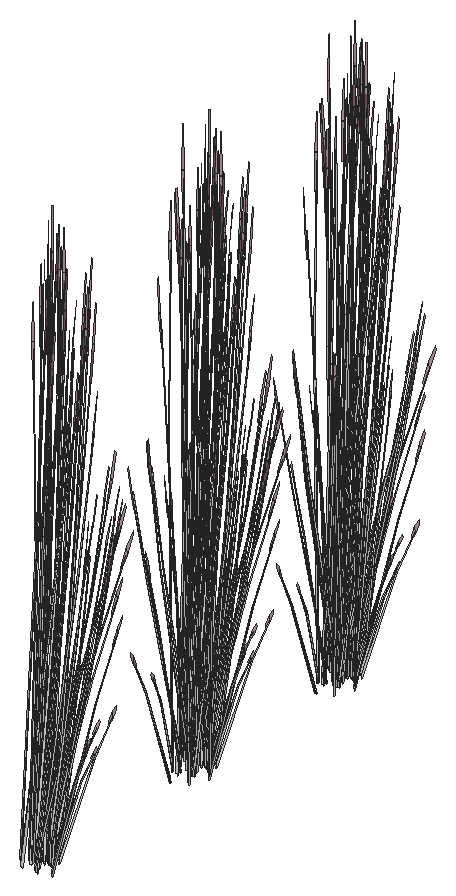
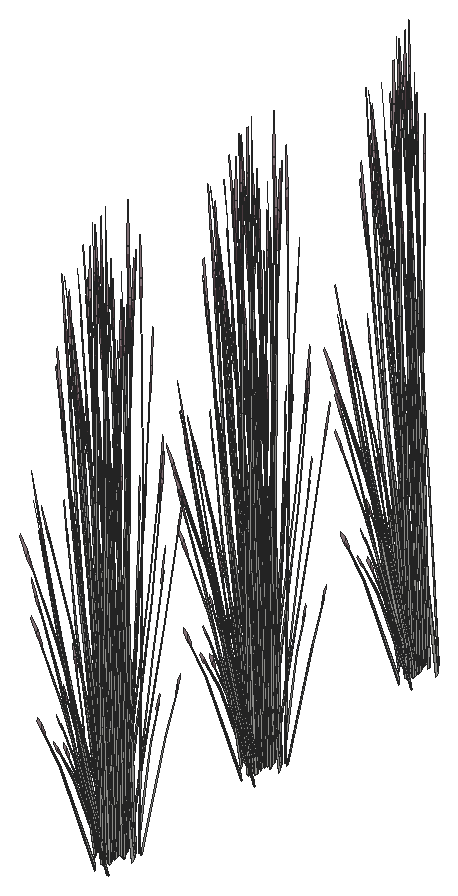
# SketchUp Ruby script. Lengths in inches.
U = 1.inch
M = Sketchup.active_model
def pt(a) = Geom::Point3d.new(a.map { |v| v * U })
def face(e, loops, mat)
  f = e.add_face(loops[0].map { |a| pt(a) })
  loops[1..].each { |l| e.add_face(l.map { |a| pt(a) }).erase! }
  f.material = f.back_material = mat if mat
  f
end
# faces: each face lists its corners as indices into pts; further lists are holes
def faces(e, pts, list, mat = nil) = list.each { |f| face(e, (f[0].is_a?(Array) ? f : [f]).map { |l| l.map { |i| pts[i] } }, mat) }
# xy, xz, yz: faces in a plane at the given z, y or x. An outline is a flat list of corners, or four numbers for a rectangle; further outlines are holes
def ring(l) = l.size == 4 ? [[l[0], l[1]], [l[2], l[1]], [l[2], l[3]], [l[0], l[3]]] : l.each_slice(2).to_a
def flat(e, list, mat, &to3) = list.each { |f| face(e, (f[0].is_a?(Array) ? f : [f]).map { |l| ring(l).map { |u, v| to3.(u, v) } }, mat) }
def xy(e, z, list, mat = nil) = flat(e, list, mat) { |x, y| [x, y, z] }
def xz(e, y, list, mat = nil) = flat(e, list, mat) { |x, z| [x, y, z] }
def yz(e, x, list, mat = nil) = flat(e, list, mat) { |y, z| [x, y, z] }
def lines(e, pts, list) = list.each { |a, b| e.add_line(pt(pts[a]), pt(pts[b])) }
# prism: a flat outline (further loops are holes) pulled along v
def prism(e, loops, v, mat = nil)
  f = face(e, loops, mat); d = Geom::Vector3d.new(v.map { |x| x * U })
  f.pushpull(f.normal.samedirection?(d) ? d.length : -d.length)
end
def box(e, o, s, mat = nil) = prism(e, [[o, [o[0] + s[0], o[1], o[2]], [o[0] + s[0], o[1] + s[1], o[2]], [o[0], o[1] + s[1], o[2]]]], [0, 0, s[2]], mat)
def at(x, y, z, deg = 0) = Geom::Transformation.translation(pt([x, y, z])) * Geom::Transformation.rotation(ORIGIN, Z_AXIS, deg.degrees)
def axes(o, x, y, z) = Geom::Transformation.new([*x, 0, *y, 0, *z, 0, *pt(o).to_a, 1])
def part(name) = M.definitions.add(name)
# library, detail: a bought-in or finely detailed component or shape, given as its bounding box
def library(name, o, s) = part(name).tap { |d| box(d.entities, o, s) }
def detail(e, o, s) = box(e.add_group.entities, o, s)
def put(e, d, t, mat = nil) = e.add_instance(d, t).tap { |i| i.material = mat if mat }
def group(e, t, mat = nil) = e.add_group.tap { |g| g.transformation = t; g.material = mat if mat }.entities
root = M.entities
M.materials.add("LightPink_Translucent").color = [144, 107, 117]
M.materials["LightPink_Translucent"].alpha = 0.75
c1 = part("blade")
p = [[2.15,0.21,22],[0,0.17,0],[0.09,0.45,0],[2.18,0.31,22],[2.29,0.31,22],[0.38,0.45,0],
  [2.48,0.24,33],[2.49,0.24,33],[2.48,0.22,33]]
faces(c1.entities,p,[[0,1,2,3],[4,5,2,3],[6,3,4,7],[8,0,3,6]])
c2 = part("seeds")
p = [[0.3,-0.1,1.38],[-0.01,-0.03,1.59],[-0.01,-0.03,0.03],[0.14,-0.07,-0.07],[0.29,-0.03,3],[0.15,0.01,3.11]]
faces(c2.entities,p,[[0,1,2,3],[1,0,4,5]],"LightPink_Translucent")
c3 = part("blade with seeds")
put(c3.entities,c1,at(0,0,0))
put(c3.entities,c2,axes([2.4,0.25,30.99],[1.5799,-0.05474,1.17369],[-0.12525,1.92788,0.29478],[-0.07173,-0.02425,1.56792]))
put(root,c3,axes([403.51,539.17,4.98],[0.31014,-0.20596,-0.71045],[0.17284,0.42397,0.08574],[0.14985,-0.04816,1.00501]))
put(root,c3,axes([402.12,538.4375,2.36],[-0.29264,0.42323,0.45755],[-0.34767,-0.3736,0.17955],[0.07055,-0.04224,1.58856]))
put(root,c3,axes([401.61,537.74,2.47],[-0.10196,0.46348,0.17642],[-0.3731,-0.13116,0.35086],[0.06445,-0.00226,1.60407]))
put(root,c3,axes([401.46,538.11,1.59],[-0.3474,0.18671,1.28929],[-0.11057,-0.53572,0.50096],[0.21332,0.00891,1.46642]))
put(root,c3,axes([402.39,538.25,2.62],[0.06809,-0.4162,0.1448],[0.33266,0.07225,-0.41347],[0.06054,0.04274,1.26744]))
put(root,c3,axes([404.17,538.84,1.49],[-0.01845,-0.0708,1.76342],[0.12793,-0.41416,-0.26939],[0.12905,-0.00596,0.30037]))
put(root,c3,axes([402.25,538.36,2.72],[-0.21202,-0.39143,0.44739],[0.32115,-0.27564,-0.21531],[0.06861,0.04843,1.43643]))
put(root,c3,axes([402.36,538.39,2.67],[0.35635,-0.30962,-0.29095],[0.23697,0.43749,-0.50002],[0.08792,0.04443,1.59708]))
put(root,c3,axes([403.78,539.21,4.53],[0.29332,0.1301,-0.35414],[-0.08555,0.37955,0.4572],[0.11809,-0.0348,0.87481]))
put(root,c3,axes([403.26,537.57,2.02],[0.33032,0.23318,-0.49651],[-0.19744,0.41812,0],[0.07523,0.05311,1.57504]))
put(root,c3,axes([402.63,538.9,2.21],[0.39487,0,0],[0,0.48281,0],[0,0,1.78407]))
put(root,c3,axes([402.74,537.76,2.47],[-0.37926,0.12378,0.17642],[-0.09365,-0.46065,0.35086],[0.03382,0.06712,1.60407]))
put(root,c3,axes([402.98,538.74,3.875],[-0.14639,0.01056,1.71376],[0.09712,-0.45778,0.13857],[0.20862,0.02831,0.73262]))
put(root,c3,axes([403.17,537.74,2.03],[0.08291,0.40636,-0.30978],[-0.32928,0.11539,0.30978],[0.06638,0.04686,1.38974]))
put(root,c3,axes([402.5,538.65,2.38],[-0.44609,-0.09826,0.49198],[0.09078,-0.55493,0.19306],[0.06519,0.05359,1.70813]))
put(root,c3,axes([402.15,540.02,2.2],[-0.11516,-0.40207,0],[0.32884,-0.1408,0],[0,0,1.54371]))
put(root,c3,axes([402.58,539.96,2.18],[0.37054,-0.15823,-0.19198],[0.1302,0.45581,0.00008],[0.0409,-0.01749,1.73897]))
put(root,c3,axes([402.62,539.1,2.21],[0.24637,0.30123,0],[-0.24637,0.30123,0],[0,0,1.69266]))
put(root,c3,axes([403.29,538.97,2.47],[-0.2773,-0.3397,0.17642],[0.27945,-0.32949,0.35086],[-0.03063,0.06937,1.60407]))
put(root,c3,axes([402.78,538.46,2.06],[0.36714,0.07646,-0.62353],[-0.07747,0.47163,-0.16365],[0.10956,0.05715,1.37633]))
put(root,c3,axes([404.4,539.28,2.77],[-0.21807,0.07699,1.1486],[0.10265,-0.31819,0.84392],[0.11568,0.02177,0.25299]))
put(root,c3,axes([402.62,538.75,2.72],[0.17124,-0.42022,0.44739],[0.35581,0.20224,-0.21531],[0,0.09687,1.43643]))
put(root,c3,axes([402.55,538.99,2.29],[0,0.53934,-0.05637],[-0.44133,0,0],[0,0.01695,1.79368]))
put(root,c3,axes([402.58,538.61,2.21],[0.21202,0.39143,-0.44739],[-0.32115,0.27564,0.21531],[0.06861,0.04843,1.43643]))
put(root,c3,axes([404.02,540.26,3.93],[-0.06755,-0.39203,-0.03492],[0.31928,-0.09013,-0.15832],[0.06667,0.02485,0.52218]))
put(root,c3,axes([403.52,538.99,2.48],[0,-0.46636,0.49651],[0.39487,0,0],[0,0.10622,1.57504]))
put(root,c3,axes([402.77,538.85,2.62],[0.32884,-0.136,0.1448],[0.11516,0.38837,-0.41347],[0,0.08547,1.26744]))
put(root,c3,axes([403.99,539.79,2.59],[-0.085,-0.1147,1.43002],[0.1106,-0.37943,-0.30754],[0.17198,0.0514,0.61141]))
put(root,c3,axes([402.47,540.21,2.2],[0.35581,0.20937,0],[-0.17124,0.43505,0],[0,0,1.74954]))
put(root,c3,axes([403.21,540.02,4.98],[0.35281,0.01123,-0.71045],[-0.0237,0.47284,0.08574],[0.14947,0.0499,1.00501]))
put(root,c3,axes([402.8125,540.4,2.48],[0.33032,-0.23318,0.49651],[0.19744,0.41812,0],[-0.07523,0.05311,1.57504]))
put(root,c3,axes([402.34,540.04,2.29],[0.15345,0.53576,-0.06012],[-0.43845,0.18773,0],[0.00536,0.01871,1.72173]))
put(root,c3,axes([403.78,539.06,2.375],[0.44133,0,0],[0,0.52122,-0.51607],[0,0.11871,1.63711]))
put(root,c3,axes([403.61,539.33,2.2],[-0.44111,-0.00373,-0.04976],[0,-0.52122,0.49943],[-0.01386,0.11865,1.58352]))
put(root,c3,axes([402.65,538.88,2.67],[0.39748,0.22252,-0.29095],[-0.19139,0.46966,-0.50002],[0.01249,0.11531,1.59708]))
put(root,c3,axes([403.42,540.22,4.53],[0.20082,0.29199,-0.35414],[-0.2293,0.2764,0.4572],[0.1165,0.04206,0.87481]))
put(root,c3,axes([403.52,539.41,2.03],[-0.24637,0.29097,-0.30978],[-0.24637,-0.29097,0.30978],[0,0.09372,1.38974]))
put(root,c3,axes([402.61,539.23,2.21],[-0.17124,0.42022,-0.44739],[-0.35581,-0.20224,0.21531],[0,0.09687,1.43643]))
put(root,c3,axes([402.62,540.43,2.33],[0.44186,0.15158,0.30756],[-0.11054,0.54181,-0.36492],[-0.07313,0.06781,1.64885]))
put(root,c3,axes([403.6875,539.42,2.02],[0,0.46636,-0.49651],[-0.39487,0,0],[0,0.10622,1.57504]))
put(root,c3,axes([402.7,539.47,3.875],[-0.1311,-0.08035,1.71376],[0.27131,-0.33708,0.13857],[0.16909,0.15206,0.73262]))
put(root,c3,axes([403.18,540.39,2.77],[-0.19872,-0.13409,1.1486],[0.2566,-0.13625,0.84392],[0.06921,0.11541,0.25299]))
put(root,c3,axes([403.24,540.88,1.49],[0.02571,-0.06733,1.76342],[0.32373,-0.19829,-0.26939],[0.09815,0.10263,0.30037]))
put(root,c3,axes([402.8125,539.36,2.09],[0.12941,0.42699,-0.69212],[-0.37279,0.15378,-0.18165],[0.0143,0.14459,1.52773]))
put(root,c3,axes([402.74,540.57,4.68],[0.34827,-0.11086,-0.51099],[0.06092,0.41983,-0.3958],[0.09354,0.12031,0.97773]))
put(root,c3,axes([403.22,541,2.67],[-0.22633,-0.01463,1.0506],[0.14947,-0.31064,0.58006],[0.08941,0.11036,0.8241]))
put(root,c3,axes([402.48,540.24,2.59],[0.00623,-0.15459,1.43002],[0.29764,-0.17268,-0.30754],[0.09188,0.18503,0.61141]))
put(root,c3,axes([401.73,540.87,1.49],[0.05712,-0.02538,1.76342],[0.34359,0.13968,-0.26939],[0.01005,0.15742,0.30037]))
put(root,c3,axes([401.96,540.77,4.68],[0.34695,0.11691,-0.51099],[-0.11892,0.40083,-0.3958],[0.03181,0.16138,0.97773]))
put(root,c3,axes([402.16,539.9375,3.875],[-0.08068,-0.14973,1.71376],[0.3728,-0.12606,0.13857],[0.08426,0.23506,0.73262]))
put(root,c3,axes([401.8,541.01,4.53],[-0.1064,0.35863,-0.35414],[-0.31043,-0.1046,0.4572],[0.02846,0.14439,0.87481]))
put(root,c3,axes([401.84,540.6875,4.98],[0.16845,0.3792,-0.71045],[-0.34676,0.21133,0.08574],[0.03939,0.18322,1.00501]))
put(root,c3,axes([402.72,558.63,2.59],[-0.10032,0.0944,1.43002],[-0.30046,-0.16522,-0.30754],[0.05569,-0.20547,0.61141]))
put(root,c3,axes([401.98,558.12,1.49],[-0.0592,0.0168,1.76342],[-0.32738,-0.18913,-0.26939],[0.00549,-0.15776,0.30037]))
put(root,c3,axes([402.97,559.33,4.98],[0.00918,-0.43138,-0.71045],[0.38672,0.02897,0.08574],[0.04081,-0.18275,1.00501]))
put(root,c3,axes([402.3,558.64,4.53],[0.1064,-0.35863,-0.35414],[0.31043,0.1046,0.4572],[-0.02846,-0.14439,0.87481]))
put(root,c3,axes([402.53,559.12,3.875],[-0.06572,0.16029,1.71376],[-0.27569,-0.33172,0.13857],[0.12437,-0.20675,0.73262]))
put(root,c3,axes([402.35,557.88,2.77],[0.04528,0.27194,1.1486],[-0.25117,-0.15062,0.84392],[0.02703,-0.13924,0.25299]))
put(root,c3,axes([402.89,559.19,4.68],[-0.25266,-0.31335,-0.51099],[0.2669,-0.27442,-0.3958],[0.03844,-0.15921,0.97773]))
put(root,c3,axes([403.13,559.07,4.53],[0.23881,-0.24554,-0.35414],[0.22606,0.28036,0.4572],[0.0344,-0.14245,0.87481]))
put(root,c3,axes([403.43,558.93,1.49],[-0.05283,-0.03674,1.76342],[-0.13569,-0.41045,-0.26939],[0.09154,-0.11138,0.30037]))
put(root,c3,axes([403.42,560.08,4.98],[0.18436,-0.36797,-0.71045],[0.32306,0.26151,0.08574],[0.11008,-0.13332,1.00501]))
put(root,c3,axes([401.43,559.01,2.375],[-0.22066,-0.46731,0],[0.36918,-0.26061,-0.51607],[0.08408,-0.05936,1.63711]))
put(root,c3,axes([403.41,559.91,4.68],[-0.09067,-0.42583,-0.51099],[0.34336,-0.07449,-0.3958],[0.0984,-0.11438,0.97773]))
put(root,c3,axes([401.73,558.94,2.02],[0.33032,-0.23318,-0.49651],[0.19744,0.41812,0],[0.07523,-0.05311,1.57504]))
put(root,c3,axes([403.69,559.75,2.59],[-0.12609,-0.01381,1.43002],[-0.12917,-0.37055,-0.30754],[0.1549,-0.10482,0.61141]))
put(root,c3,axes([402.12,559.9,2.06],[0.23773,-0.35053,-0.62353],[0.29532,0.31785,-0.16365],[0.09526,-0.08744,1.37633]))
put(root,c3,axes([403.84,559.06,2.77],[-0.11756,0.2374,1.1486],[-0.10105,-0.31895,0.84392],[0.09709,-0.07992,0.25299]))
put(root,c3,axes([403.67,559.96,4.53],[0.30722,-0.06665,-0.35414],[0.08112,0.381,0.4572],[0.08804,-0.10234,0.87481]))
put(root,c3,axes([401.71,560.51,2.21],[0.17124,-0.42022,-0.44739],[0.35581,0.20224,0.21531],[0,-0.09687,1.43643]))
put(root,c3,axes([401.86,560.3,2.67],[-0.04113,-0.53214,-0.29095],[0.42835,-0.03218,-0.50002],[0.07543,-0.07088,1.59708]))
put(root,c3,axes([401.81,559.125,2.03],[0.32928,0.11539,-0.30978],[-0.08291,0.40636,0.30978],[0.06638,-0.04686,1.38974]))
put(root,c3,axes([401.92,560.72,2.43],[0.39767,0.22603,0.24065],[-0.19139,0.46966,0.50002],[0,-0.10827,1.60543]))
put(root,c3,axes([401.79,560.4,2.72],[-0.38326,0.02879,0.44739],[-0.03466,-0.47788,-0.21531],[0.06861,-0.04843,1.43643]))
put(root,c3,axes([403.57,560.86,4.68],[0.09562,-0.42421,-0.51099],[0.32782,0.1454,-0.3958],[0.13199,-0.0389,0.97773]))
put(root,c3,axes([403.06,559.13,2.375],[0.22066,-0.46731,0],[0.36918,0.26061,-0.51607],[0.08408,0.05936,1.63711]))
put(root,c3,axes([401.78,560.58,2.36],[0.15345,0.52148,0.45755],[-0.43845,0.18134,0.17955],[0.00536,-0.09582,1.58856]))
put(root,c3,axes([403.92,560.98,1.98],[-0.22732,0.05597,1.41583],[-0.03618,-0.44548,0.08104],[0.15921,-0.06743,0.80566]))
put(root,c3,axes([404.34,560.58,2.26],[-0.21881,-0.29821,-0.06488],[0.23965,-0.27324,-0.29416],[0.0679,-0.01924,0.97024]))
put(root,c3,axes([402.33,560.62,2.21],[0,-0.53961,0],[0.44133,0,0],[0,0,1.79456]))
put(root,c3,axes([402.87,559.375,2.48],[-0.33032,-0.23318,0.49651],[0.19744,-0.41812,0],[0.07523,0.05311,1.57504]))
put(root,c3,axes([403.51,561.01,4.98],[0.31014,-0.20596,-0.71045],[0.17284,0.42397,0.08574],[0.14985,-0.04816,1.00501]))
put(root,c3,axes([402.12,560.28,2.36],[-0.29264,0.42323,0.45755],[-0.34767,-0.3736,0.17955],[0.07055,-0.04224,1.58856]))
put(root,c3,axes([401.61,559.58,2.47],[-0.10196,0.46348,0.17642],[-0.3731,-0.13116,0.35086],[0.06445,-0.00226,1.60407]))
put(root,c3,axes([401.46,559.96,1.59],[-0.3474,0.18671,1.28929],[-0.11057,-0.53572,0.50096],[0.21332,0.00891,1.46642]))
put(root,c3,axes([402.39,560.1,2.62],[0.06809,-0.4162,0.1448],[0.33266,0.07225,-0.41347],[0.06054,0.04274,1.26744]))
put(root,c3,axes([404.17,560.6875,1.49],[-0.01845,-0.0708,1.76342],[0.12793,-0.41416,-0.26939],[0.12905,-0.00596,0.30037]))
put(root,c3,axes([402.25,560.21,2.72],[-0.21202,-0.39143,0.44739],[0.32115,-0.27564,-0.21531],[0.06861,0.04843,1.43643]))
put(root,c3,axes([402.36,560.23,2.67],[0.35635,-0.30962,-0.29095],[0.23697,0.43749,-0.50002],[0.08792,0.04443,1.59708]))
put(root,c3,axes([403.78,561.05,4.53],[0.29332,0.1301,-0.35414],[-0.08555,0.37955,0.4572],[0.11809,-0.0348,0.87481]))
put(root,c3,axes([403.26,559.41,2.02],[0.33032,0.23318,-0.49651],[-0.19744,0.41812,0],[0.07523,0.05311,1.57504]))
put(root,c3,axes([402.63,560.74,2.21],[0.39487,0,0],[0,0.48281,0],[0,0,1.78407]))
put(root,c3,axes([402.74,559.61,2.47],[-0.37926,0.12378,0.17642],[-0.09365,-0.46065,0.35086],[0.03382,0.06712,1.60407]))
put(root,c3,axes([402.98,560.58,3.875],[-0.14639,0.01056,1.71376],[0.09712,-0.45778,0.13857],[0.20862,0.02831,0.73262]))
put(root,c3,axes([403.17,559.59,2.03],[0.08291,0.40636,-0.30978],[-0.32928,0.11539,0.30978],[0.06638,0.04686,1.38974]))
put(root,c3,axes([402.5,560.5,2.38],[-0.44609,-0.09826,0.49198],[0.09078,-0.55493,0.19306],[0.06519,0.05359,1.70813]))
put(root,c3,axes([402.15,561.87,2.2],[-0.11516,-0.40207,0],[0.32884,-0.1408,0],[0,0,1.54371]))
put(root,c3,axes([402.58,561.81,2.18],[0.37054,-0.15823,-0.19198],[0.1302,0.45581,0.00008],[0.0409,-0.01749,1.73897]))
put(root,c3,axes([402.62,560.95,2.21],[0.24637,0.30123,0],[-0.24637,0.30123,0],[0,0,1.69266]))
put(root,c3,axes([403.29,560.82,2.47],[-0.2773,-0.3397,0.17642],[0.27945,-0.32949,0.35086],[-0.03063,0.06937,1.60407]))
put(root,c3,axes([402.78,560.3,2.06],[0.36714,0.07646,-0.62353],[-0.07747,0.47163,-0.16365],[0.10956,0.05715,1.37633]))
put(root,c3,axes([404.4,561.13,2.77],[-0.21807,0.07699,1.1486],[0.10265,-0.31819,0.84392],[0.11568,0.02177,0.25299]))
put(root,c3,axes([402.62,560.6,2.72],[0.17124,-0.42022,0.44739],[0.35581,0.20224,-0.21531],[0,0.09687,1.43643]))
put(root,c3,axes([402.55,560.84,2.29],[0,0.53934,-0.05637],[-0.44133,0,0],[0,0.01695,1.79368]))
put(root,c3,axes([402.58,560.45,2.21],[0.21202,0.39143,-0.44739],[-0.32115,0.27564,0.21531],[0.06861,0.04843,1.43643]))
put(root,c3,axes([404.02,562.11,3.93],[-0.06755,-0.39203,-0.03492],[0.31928,-0.09013,-0.15832],[0.06667,0.02485,0.52218]))
put(root,c3,axes([403.52,560.83,2.48],[0,-0.46636,0.49651],[0.39487,0,0],[0,0.10622,1.57504]))
put(root,c3,axes([402.77,560.69,2.62],[0.32884,-0.136,0.1448],[0.11516,0.38837,-0.41347],[0,0.08547,1.26744]))
put(root,c3,axes([403.99,561.64,2.59],[-0.085,-0.1147,1.43002],[0.1106,-0.37943,-0.30754],[0.17198,0.0514,0.61141]))
put(root,c3,axes([402.47,562.06,2.2],[0.35581,0.20937,0],[-0.17124,0.43505,0],[0,0,1.74954]))
put(root,c3,axes([403.21,561.87,4.98],[0.35281,0.01123,-0.71045],[-0.0237,0.47284,0.08574],[0.14947,0.0499,1.00501]))
put(root,c3,axes([402.8125,562.25,2.48],[0.33032,-0.23318,0.49651],[0.19744,0.41812,0],[-0.07523,0.05311,1.57504]))
put(root,c3,axes([402.34,561.88,2.29],[0.15345,0.53576,-0.06012],[-0.43845,0.18773,0],[0.00536,0.01871,1.72173]))
put(root,c3,axes([403.78,560.91,2.375],[0.44133,0,0],[0,0.52122,-0.51607],[0,0.11871,1.63711]))
put(root,c3,axes([403.61,561.18,2.2],[-0.44111,-0.00373,-0.04976],[0,-0.52122,0.49943],[-0.01386,0.11865,1.58352]))
put(root,c3,axes([402.65,560.72,2.67],[0.39748,0.22252,-0.29095],[-0.19139,0.46966,-0.50002],[0.01249,0.11531,1.59708]))
put(root,c3,axes([403.42,562.0625,4.53],[0.20082,0.29199,-0.35414],[-0.2293,0.2764,0.4572],[0.1165,0.04206,0.87481]))
put(root,c3,axes([403.52,561.25,2.03],[-0.24637,0.29097,-0.30978],[-0.24637,-0.29097,0.30978],[0,0.09372,1.38974]))
put(root,c3,axes([402.61,561.07,2.21],[-0.17124,0.42022,-0.44739],[-0.35581,-0.20224,0.21531],[0,0.09687,1.43643]))
put(root,c3,axes([402.62,562.28,2.33],[0.44186,0.15158,0.30756],[-0.11054,0.54181,-0.36492],[-0.07313,0.06781,1.64885]))
put(root,c3,axes([403.6875,561.26,2.02],[0,0.46636,-0.49651],[-0.39487,0,0],[0,0.10622,1.57504]))
put(root,c3,axes([402.7,561.32,3.875],[-0.1311,-0.08035,1.71376],[0.27131,-0.33708,0.13857],[0.16909,0.15206,0.73262]))
put(root,c3,axes([403.18,562.23,2.77],[-0.19872,-0.13409,1.1486],[0.2566,-0.13625,0.84392],[0.06921,0.11541,0.25299]))
put(root,c3,axes([403.24,562.73,1.49],[0.02571,-0.06733,1.76342],[0.32373,-0.19829,-0.26939],[0.09815,0.10263,0.30037]))
put(root,c3,axes([402.8125,561.2,2.09],[0.12941,0.42699,-0.69212],[-0.37279,0.15378,-0.18165],[0.0143,0.14459,1.52773]))
put(root,c3,axes([402.74,562.42,4.68],[0.34827,-0.11086,-0.51099],[0.06092,0.41983,-0.3958],[0.09354,0.12031,0.97773]))
put(root,c3,axes([403.22,562.84,2.67],[-0.22633,-0.01463,1.0506],[0.14947,-0.31064,0.58006],[0.08941,0.11036,0.8241]))
put(root,c3,axes([402.48,562.09,2.59],[0.00623,-0.15459,1.43002],[0.29764,-0.17268,-0.30754],[0.09188,0.18503,0.61141]))
put(root,c3,axes([401.73,562.71,1.49],[0.05712,-0.02538,1.76342],[0.34359,0.13968,-0.26939],[0.01005,0.15742,0.30037]))
put(root,c3,axes([401.96,562.61,4.68],[0.34695,0.11691,-0.51099],[-0.11892,0.40083,-0.3958],[0.03181,0.16138,0.97773]))
put(root,c3,axes([402.16,561.78,3.875],[-0.08068,-0.14973,1.71376],[0.3728,-0.12606,0.13857],[0.08426,0.23506,0.73262]))
put(root,c3,axes([401.8,562.86,4.53],[-0.1064,0.35863,-0.35414],[-0.31043,-0.1046,0.4572],[0.02846,0.14439,0.87481]))
put(root,c3,axes([401.84,562.53,4.98],[0.16845,0.3792,-0.71045],[-0.34676,0.21133,0.08574],[0.03939,0.18322,1.00501]))
put(root,c3,axes([402.72,578.9,2.59],[-0.10032,0.0944,1.43002],[-0.30046,-0.16522,-0.30754],[0.05569,-0.20547,0.61141]))
put(root,c3,axes([401.98,578.39,1.49],[-0.0592,0.0168,1.76342],[-0.32738,-0.18913,-0.26939],[0.00549,-0.15776,0.30037]))
put(root,c3,axes([402.97,579.6,4.98],[0.00918,-0.43138,-0.71045],[0.38672,0.02897,0.08574],[0.04081,-0.18275,1.00501]))
put(root,c3,axes([402.3,578.91,4.53],[0.1064,-0.35863,-0.35414],[0.31043,0.1046,0.4572],[-0.02846,-0.14439,0.87481]))
put(root,c3,axes([402.53,579.38,3.875],[-0.06572,0.16029,1.71376],[-0.27569,-0.33172,0.13857],[0.12437,-0.20675,0.73262]))
put(root,c3,axes([402.35,578.15,2.77],[0.04528,0.27194,1.1486],[-0.25117,-0.15062,0.84392],[0.02703,-0.13924,0.25299]))
put(root,c3,axes([402.89,579.46,4.68],[-0.25266,-0.31335,-0.51099],[0.2669,-0.27442,-0.3958],[0.03844,-0.15921,0.97773]))
put(root,c3,axes([403.13,579.34,4.53],[0.23881,-0.24554,-0.35414],[0.22606,0.28036,0.4572],[0.0344,-0.14245,0.87481]))
put(root,c3,axes([403.43,579.19,1.49],[-0.05283,-0.03674,1.76342],[-0.13569,-0.41045,-0.26939],[0.09154,-0.11138,0.30037]))
put(root,c3,axes([403.42,580.35,4.98],[0.18436,-0.36797,-0.71045],[0.32306,0.26151,0.08574],[0.11008,-0.13332,1.00501]))
put(root,c3,axes([401.43,579.28,2.375],[-0.22066,-0.46731,0],[0.36918,-0.26061,-0.51607],[0.08408,-0.05936,1.63711]))
put(root,c3,axes([403.41,580.18,4.68],[-0.09067,-0.42583,-0.51099],[0.34336,-0.07449,-0.3958],[0.0984,-0.11438,0.97773]))
put(root,c3,axes([401.73,579.21,2.02],[0.33032,-0.23318,-0.49651],[0.19744,0.41812,0],[0.07523,-0.05311,1.57504]))
put(root,c3,axes([403.69,580.01,2.59],[-0.12609,-0.01381,1.43002],[-0.12917,-0.37055,-0.30754],[0.1549,-0.10482,0.61141]))
put(root,c3,axes([402.12,580.16,2.06],[0.23773,-0.35053,-0.62353],[0.29532,0.31785,-0.16365],[0.09526,-0.08744,1.37633]))
put(root,c3,axes([403.84,579.33,2.77],[-0.11756,0.2374,1.1486],[-0.10105,-0.31895,0.84392],[0.09709,-0.07992,0.25299]))
put(root,c3,axes([403.67,580.22,4.53],[0.30722,-0.06665,-0.35414],[0.08112,0.381,0.4572],[0.08804,-0.10234,0.87481]))
put(root,c3,axes([401.71,580.78,2.21],[0.17124,-0.42022,-0.44739],[0.35581,0.20224,0.21531],[0,-0.09687,1.43643]))
put(root,c3,axes([401.86,580.57,2.67],[-0.04113,-0.53214,-0.29095],[0.42835,-0.03218,-0.50002],[0.07543,-0.07088,1.59708]))
put(root,c3,axes([401.81,579.39,2.03],[0.32928,0.11539,-0.30978],[-0.08291,0.40636,0.30978],[0.06638,-0.04686,1.38974]))
put(root,c3,axes([401.92,580.99,2.43],[0.39767,0.22603,0.24065],[-0.19139,0.46966,0.50002],[0,-0.10827,1.60543]))
put(root,c3,axes([401.79,580.67,2.72],[-0.38326,0.02879,0.44739],[-0.03466,-0.47788,-0.21531],[0.06861,-0.04843,1.43643]))
put(root,c3,axes([403.57,581.125,4.68],[0.09562,-0.42421,-0.51099],[0.32782,0.1454,-0.3958],[0.13199,-0.0389,0.97773]))
put(root,c3,axes([403.06,579.4,2.375],[0.22066,-0.46731,0],[0.36918,0.26061,-0.51607],[0.08408,0.05936,1.63711]))
put(root,c3,axes([401.78,580.84,2.36],[0.15345,0.52148,0.45755],[-0.43845,0.18134,0.17955],[0.00536,-0.09582,1.58856]))
put(root,c3,axes([403.92,581.24,1.98],[-0.22732,0.05597,1.41583],[-0.03618,-0.44548,0.08104],[0.15921,-0.06743,0.80566]))
put(root,c3,axes([404.34,580.85,2.26],[-0.21881,-0.29821,-0.06488],[0.23965,-0.27324,-0.29416],[0.0679,-0.01924,0.97024]))
put(root,c3,axes([402.33,580.89,2.21],[0,-0.53961,0],[0.44133,0,0],[0,0,1.79456]))
put(root,c3,axes([402.87,579.64,2.48],[-0.33032,-0.23318,0.49651],[0.19744,-0.41812,0],[0.07523,0.05311,1.57504]))
put(root,c3,axes([403.51,581.28,4.98],[0.31014,-0.20596,-0.71045],[0.17284,0.42397,0.08574],[0.14985,-0.04816,1.00501]))
put(root,c3,axes([402.12,580.55,2.36],[-0.29264,0.42323,0.45755],[-0.34767,-0.3736,0.17955],[0.07055,-0.04224,1.58856]))
put(root,c3,axes([401.61,579.85,2.47],[-0.10196,0.46348,0.17642],[-0.3731,-0.13116,0.35086],[0.06445,-0.00226,1.60407]))
put(root,c3,axes([401.46,580.23,1.59],[-0.3474,0.18671,1.28929],[-0.11057,-0.53572,0.50096],[0.21332,0.00891,1.46642]))
put(root,c3,axes([402.39,580.37,2.62],[0.06809,-0.4162,0.1448],[0.33266,0.07225,-0.41347],[0.06054,0.04274,1.26744]))
put(root,c3,axes([404.17,580.95,1.49],[-0.01845,-0.0708,1.76342],[0.12793,-0.41416,-0.26939],[0.12905,-0.00596,0.30037]))
put(root,c3,axes([402.25,580.48,2.72],[-0.21202,-0.39143,0.44739],[0.32115,-0.27564,-0.21531],[0.06861,0.04843,1.43643]))
put(root,c3,axes([402.36,580.5,2.67],[0.35635,-0.30962,-0.29095],[0.23697,0.43749,-0.50002],[0.08792,0.04443,1.59708]))
put(root,c3,axes([403.78,581.32,4.53],[0.29332,0.1301,-0.35414],[-0.08555,0.37955,0.4572],[0.11809,-0.0348,0.87481]))
put(root,c3,axes([403.26,579.68,2.02],[0.33032,0.23318,-0.49651],[-0.19744,0.41812,0],[0.07523,0.05311,1.57504]))
put(root,c3,axes([402.63,581.01,2.21],[0.39487,0,0],[0,0.48281,0],[0,0,1.78407]))
put(root,c3,axes([402.74,579.88,2.47],[-0.37926,0.12378,0.17642],[-0.09365,-0.46065,0.35086],[0.03382,0.06712,1.60407]))
put(root,c3,axes([402.98,580.85,3.875],[-0.14639,0.01056,1.71376],[0.09712,-0.45778,0.13857],[0.20862,0.02831,0.73262]))
put(root,c3,axes([403.17,579.85,2.03],[0.08291,0.40636,-0.30978],[-0.32928,0.11539,0.30978],[0.06638,0.04686,1.38974]))
put(root,c3,axes([402.5,580.76,2.38],[-0.44609,-0.09826,0.49198],[0.09078,-0.55493,0.19306],[0.06519,0.05359,1.70813]))
put(root,c3,axes([402.15,582.13,2.2],[-0.11516,-0.40207,0],[0.32884,-0.1408,0],[0,0,1.54371]))
put(root,c3,axes([402.58,582.08,2.18],[0.37054,-0.15823,-0.19198],[0.1302,0.45581,0.00008],[0.0409,-0.01749,1.73897]))
put(root,c3,axes([402.62,581.22,2.21],[0.24637,0.30123,0],[-0.24637,0.30123,0],[0,0,1.69266]))
put(root,c3,axes([403.29,581.08,2.47],[-0.2773,-0.3397,0.17642],[0.27945,-0.32949,0.35086],[-0.03063,0.06937,1.60407]))
put(root,c3,axes([402.78,580.57,2.06],[0.36714,0.07646,-0.62353],[-0.07747,0.47163,-0.16365],[0.10956,0.05715,1.37633]))
put(root,c3,axes([404.4,581.4,2.77],[-0.21807,0.07699,1.1486],[0.10265,-0.31819,0.84392],[0.11568,0.02177,0.25299]))
put(root,c3,axes([402.62,580.86,2.72],[0.17124,-0.42022,0.44739],[0.35581,0.20224,-0.21531],[0,0.09687,1.43643]))
put(root,c3,axes([402.55,581.1,2.29],[0,0.53934,-0.05637],[-0.44133,0,0],[0,0.01695,1.79368]))
put(root,c3,axes([402.58,580.72,2.21],[0.21202,0.39143,-0.44739],[-0.32115,0.27564,0.21531],[0.06861,0.04843,1.43643]))
put(root,c3,axes([404.02,582.375,3.93],[-0.06755,-0.39203,-0.03492],[0.31928,-0.09013,-0.15832],[0.06667,0.02485,0.52218]))
put(root,c3,axes([403.52,581.1,2.48],[0,-0.46636,0.49651],[0.39487,0,0],[0,0.10622,1.57504]))
put(root,c3,axes([402.77,580.96,2.62],[0.32884,-0.136,0.1448],[0.11516,0.38837,-0.41347],[0,0.08547,1.26744]))
put(root,c3,axes([403.99,581.91,2.59],[-0.085,-0.1147,1.43002],[0.1106,-0.37943,-0.30754],[0.17198,0.0514,0.61141]))
put(root,c3,axes([402.47,582.32,2.2],[0.35581,0.20937,0],[-0.17124,0.43505,0],[0,0,1.74954]))
put(root,c3,axes([403.21,582.14,4.98],[0.35281,0.01123,-0.71045],[-0.0237,0.47284,0.08574],[0.14947,0.0499,1.00501]))
put(root,c3,axes([402.8125,582.52,2.48],[0.33032,-0.23318,0.49651],[0.19744,0.41812,0],[-0.07523,0.05311,1.57504]))
put(root,c3,axes([402.34,582.15,2.29],[0.15345,0.53576,-0.06012],[-0.43845,0.18773,0],[0.00536,0.01871,1.72173]))
put(root,c3,axes([403.78,581.18,2.375],[0.44133,0,0],[0,0.52122,-0.51607],[0,0.11871,1.63711]))
put(root,c3,axes([403.61,581.45,2.2],[-0.44111,-0.00373,-0.04976],[0,-0.52122,0.49943],[-0.01386,0.11865,1.58352]))
put(root,c3,axes([402.65,580.99,2.67],[0.39748,0.22252,-0.29095],[-0.19139,0.46966,-0.50002],[0.01249,0.11531,1.59708]))
put(root,c3,axes([403.42,582.33,4.53],[0.20082,0.29199,-0.35414],[-0.2293,0.2764,0.4572],[0.1165,0.04206,0.87481]))
put(root,c3,axes([403.52,581.52,2.03],[-0.24637,0.29097,-0.30978],[-0.24637,-0.29097,0.30978],[0,0.09372,1.38974]))
put(root,c3,axes([402.61,581.34,2.21],[-0.17124,0.42022,-0.44739],[-0.35581,-0.20224,0.21531],[0,0.09687,1.43643]))
put(root,c3,axes([402.62,582.55,2.33],[0.44186,0.15158,0.30756],[-0.11054,0.54181,-0.36492],[-0.07313,0.06781,1.64885]))
put(root,c3,axes([403.6875,581.53,2.02],[0,0.46636,-0.49651],[-0.39487,0,0],[0,0.10622,1.57504]))
put(root,c3,axes([402.7,581.58,3.875],[-0.1311,-0.08035,1.71376],[0.27131,-0.33708,0.13857],[0.16909,0.15206,0.73262]))
put(root,c3,axes([403.18,582.5,2.77],[-0.19872,-0.13409,1.1486],[0.2566,-0.13625,0.84392],[0.06921,0.11541,0.25299]))
put(root,c3,axes([403.24,583,1.49],[0.02571,-0.06733,1.76342],[0.32373,-0.19829,-0.26939],[0.09815,0.10263,0.30037]))
put(root,c3,axes([402.8125,581.47,2.09],[0.12941,0.42699,-0.69212],[-0.37279,0.15378,-0.18165],[0.0143,0.14459,1.52773]))
put(root,c3,axes([402.74,582.68,4.68],[0.34827,-0.11086,-0.51099],[0.06092,0.41983,-0.3958],[0.09354,0.12031,0.97773]))
put(root,c3,axes([403.22,583.11,2.67],[-0.22633,-0.01463,1.0506],[0.14947,-0.31064,0.58006],[0.08941,0.11036,0.8241]))
put(root,c3,axes([402.48,582.36,2.59],[0.00623,-0.15459,1.43002],[0.29764,-0.17268,-0.30754],[0.09188,0.18503,0.61141]))
put(root,c3,axes([401.73,582.98,1.49],[0.05712,-0.02538,1.76342],[0.34359,0.13968,-0.26939],[0.01005,0.15742,0.30037]))
